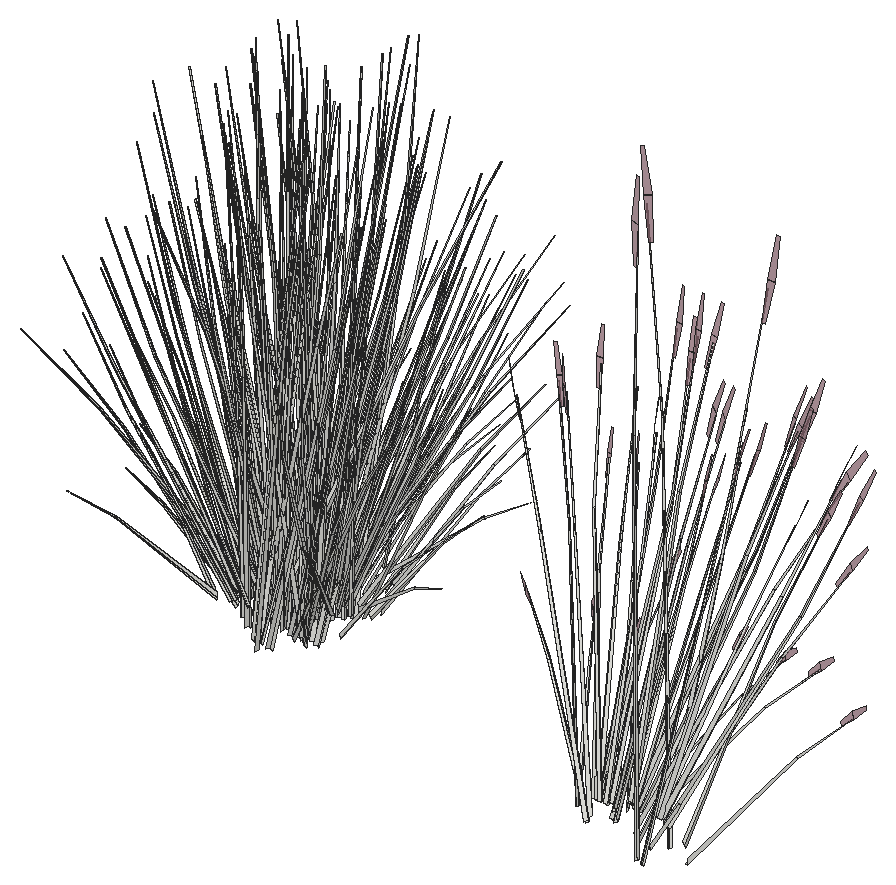
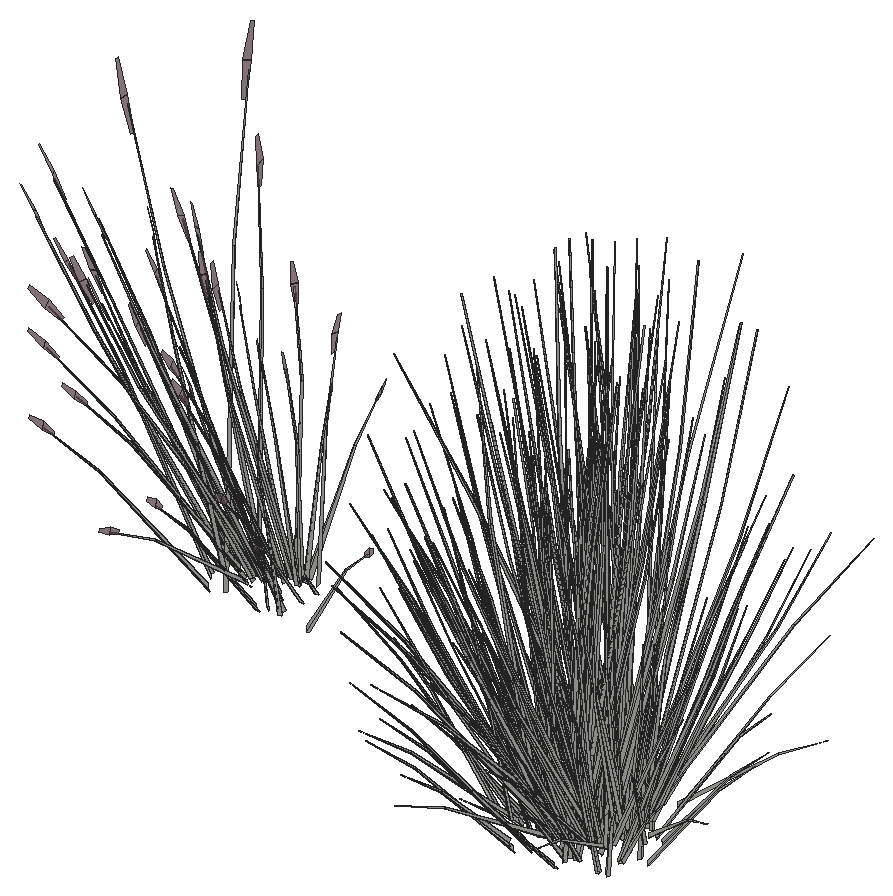
# SketchUp Ruby script. Lengths in inches.
U = 1.inch
M = Sketchup.active_model
def pt(a) = Geom::Point3d.new(a.map { |v| v * U })
def face(e, loops, mat)
  f = e.add_face(loops[0].map { |a| pt(a) })
  loops[1..].each { |l| e.add_face(l.map { |a| pt(a) }).erase! }
  f.material = f.back_material = mat if mat
  f
end
# faces: each face lists its corners as indices into pts; further lists are holes
def faces(e, pts, list, mat = nil) = list.each { |f| face(e, (f[0].is_a?(Array) ? f : [f]).map { |l| l.map { |i| pts[i] } }, mat) }
# xy, xz, yz: faces in a plane at the given z, y or x. An outline is a flat list of corners, or four numbers for a rectangle; further outlines are holes
def ring(l) = l.size == 4 ? [[l[0], l[1]], [l[2], l[1]], [l[2], l[3]], [l[0], l[3]]] : l.each_slice(2).to_a
def flat(e, list, mat, &to3) = list.each { |f| face(e, (f[0].is_a?(Array) ? f : [f]).map { |l| ring(l).map { |u, v| to3.(u, v) } }, mat) }
def xy(e, z, list, mat = nil) = flat(e, list, mat) { |x, y| [x, y, z] }
def xz(e, y, list, mat = nil) = flat(e, list, mat) { |x, z| [x, y, z] }
def yz(e, x, list, mat = nil) = flat(e, list, mat) { |y, z| [x, y, z] }
def lines(e, pts, list) = list.each { |a, b| e.add_line(pt(pts[a]), pt(pts[b])) }
# prism: a flat outline (further loops are holes) pulled along v
def prism(e, loops, v, mat = nil)
  f = face(e, loops, mat); d = Geom::Vector3d.new(v.map { |x| x * U })
  f.pushpull(f.normal.samedirection?(d) ? d.length : -d.length)
end
def box(e, o, s, mat = nil) = prism(e, [[o, [o[0] + s[0], o[1], o[2]], [o[0] + s[0], o[1] + s[1], o[2]], [o[0], o[1] + s[1], o[2]]]], [0, 0, s[2]], mat)
def at(x, y, z, deg = 0) = Geom::Transformation.translation(pt([x, y, z])) * Geom::Transformation.rotation(ORIGIN, Z_AXIS, deg.degrees)
def axes(o, x, y, z) = Geom::Transformation.new([*x, 0, *y, 0, *z, 0, *pt(o).to_a, 1])
def part(name) = M.definitions.add(name)
# library, detail: a bought-in or finely detailed component or shape, given as its bounding box
def library(name, o, s) = part(name).tap { |d| box(d.entities, o, s) }
def detail(e, o, s) = box(e.add_group.entities, o, s)
def put(e, d, t, mat = nil) = e.add_instance(d, t).tap { |i| i.material = mat if mat }
def group(e, t, mat = nil) = e.add_group.tap { |g| g.transformation = t; g.material = mat if mat }.entities
root = M.entities
M.materials.add("LightPink_Translucent").color = [144, 107, 117]
M.materials["LightPink_Translucent"].alpha = 0.75
c1 = part("blade")
p = [[2.15,0.21,22],[0,0.17,0],[0.09,0.45,0],[2.18,0.31,22],[2.29,0.31,22],[0.38,0.45,0],
  [2.48,0.24,33],[2.49,0.24,33],[2.48,0.22,33]]
faces(c1.entities,p,[[0,1,2,3],[4,5,2,3],[6,3,4,7],[8,0,3,6]])
c2 = part("seeds")
p = [[0.3,-0.1,1.38],[-0.01,-0.03,1.59],[-0.01,-0.03,0.03],[0.14,-0.07,-0.07],[0.29,-0.03,3],[0.15,0.01,3.11]]
faces(c2.entities,p,[[0,1,2,3],[1,0,4,5]],"LightPink_Translucent")
c3 = part("blade with seeds")
put(c3.entities,c1,at(0,0,0))
put(c3.entities,c2,axes([2.4,0.25,30.99],[1.5799,-0.05474,1.17369],[-0.12525,1.92788,0.29478],[-0.07173,-0.02425,1.56792]))
c4 = part("blade with seeds\#1")
put(c4.entities,c1,at(0,0,0))
put(root,c3,axes([267.38,266.44,17.27],[0.73026,-0.88648,-0.1216],[1.05755,0.51071,-0.67495],[0.36761,0.25045,1.02557]))
put(root,c4,axes([224.3,276.92,16.28],[-0.8363,-0.68892,-0.10962],[0.4818,-0.99769,-0.60845],[0.23628,-0.3468,0.92453]))
put(root,c3,axes([262.1,263.23,16.11],[0.30609,-0.31822,1.71376],[0.77286,0.85893,0.13857],[-0.53009,0.39116,0.73262]))
put(root,c3,axes([261.13,264.16,16.92],[0.31482,0.94565,-0.51099],[-1.19224,0.16542,-0.3958],[-0.34166,0.254,0.97773]))
put(root,c4,axes([218.74,280.28,13.18],[0.39117,1.13797,1.16227],[-1.12236,0.3622,0.45161],[0.01867,-0.69878,1.32195]))
put(root,c3,axes([262.5625,265.24,17.29],[0.82919,-0.54528,0.35414],[0.78493,0.62262,-0.4572],[-0.11943,0.31634,0.87481]))
put(root,c3,axes([268.77,266.35,14.61],[0.7662,1.03778,0],[-1.28187,0.57875,-0.51607],[-0.29196,0.13181,1.63711]))
put(root,c4,axes([219.2,273.87,16.29],[0.13963,1.00636,0.31925],[-0.79822,0.26574,-0.41216],[-0.2144,-0.28839,0.78863]))
put(root,c3,axes([266.42,267.18,16.95],[0.00363,-0.12539,1.77383],[1.0502,-0.55319,-0.16761],[0.36479,0.19745,0.31391]))
put(root,c4,axes([224.77,274.52,14.14],[-0.03064,0.74138,0.9471],[-0.6508,-0.48961,0.52291],[0.23122,-0.29288,0.74292]))
put(root,c3,axes([270,266.7,13.73],[0.08928,-0.14952,1.76342],[1.12407,-0.44035,-0.26939],[0.34078,0.22791,0.30037]))
put(root,c3,axes([268.12,262.24,15.08],[-0.03348,-0.97511,1.41272],[1.51511,0.25277,0.59816],[-0.35835,0.53357,1.3335]))
put(root,c3,axes([268.51,263.3,14.33],[0.44936,0.94823,-0.69212],[-1.29441,0.3415,-0.18165],[0.04967,0.32109,1.52773]))
put(root,c3,axes([261.8125,265.74,16.97],[-1.00708,-0.04826,0.0643],[0.02761,-0.72867,0.50621],[-0.10538,0.27912,0.77189]))
put(root,c4,axes([216.97,276.76,15.23],[0.33582,0.21526,1.54493],[-0.69497,0.90306,0.12492],[-0.43315,-0.40739,0.66044]))
put(root,c3,axes([259.67,266.57,13.73],[0.16438,0.10347,1.76342],[0.27873,0.95868,-0.26939],[-0.36432,0.20444,0.30037]))
put(root,c3,axes([262.13,265.8,16.97],[-0.87265,-0.70663,0.48003],[0.92674,-0.60943,0.3958],[-0.16097,0.33153,0.9933]))
put(root,c3,axes([268.24,266,16.92],[1.20928,-0.24619,-0.51099],[0.21154,0.93233,-0.3958],[0.32481,0.26718,0.97773]))
put(root,c3,axes([264.89,266.14,17.29],[0.36946,-0.79643,0.35414],[1.07787,0.23229,-0.4572],[0.09883,0.32066,0.87481]))
put(root,c4,axes([220.73,272.66,13.88],[0,-1.44565,0],[1.09198,0,-0.46523],[0.24871,0,1.47583]))
put(root,c4,axes([219.3125,277.33,14.14],[-0.64866,-1.16728,-0.26229],[0.91655,-0.77622,-0.45076],[0.09308,-0.288,1.43974]))
put(root,c4,axes([217.95,274.69,13.57],[0.85134,-0.27158,-0.27926],[0.24175,1.0786,0.27926],[0.09817,-0.21744,1.25283]))
put(root,c3,axes([269.91,266.95,14.9],[-0.78586,-0.03248,1.0506],[0.51898,-0.68985,0.58006],[0.31045,0.24509,0.8241]))
put(root,c4,axes([223.5,274.63,14.23],[-0.28093,0.65095,1.03545],[-0.28545,-0.84053,0.76078],[0.2418,-0.22671,0.22807]))
put(root,c3,axes([267.65,266.76,16.97],[-0.55698,0.6579,0.0643],[-0.79316,-0.38303,0.50621],[0.25643,0.21093,0.77189]))
put(root,c4,axes([216.02,273.57,15.99],[-0.19445,0.01116,1.57709],[-0.562,0.94258,-0.24942],[-0.34067,-0.14573,0.12648]))
put(root,c4,axes([217.08,274.82,16.01],[0.66663,-0.82326,0.43274],[0.57493,0.87428,0.35681],[-0.31276,-0.15186,0.89544]))
put(root,c3,axes([266.34,268.98,17.88],[0.84686,-0.59414,-0.06488],[0.77596,0.65071,-0.29416],[0.05463,0.18438,0.97024]))
put(root,c4,axes([223.2,276.95,14.08],[-0.32388,-0.0204,1.28914],[-0.36177,-0.97496,-0.27724],[0.38765,-0.30097,0.55117]))
put(root,c4,axes([218.61,278.11,13.6],[-0.73437,-0.77871,-0.5621],[0.66591,-0.96736,-0.14753],[-0.18319,-0.31204,1.24074]))
put(root,c4,axes([217.15,274.52,16],[0.04552,-0.95007,0.05797],[0.68742,0.02605,0.45634],[-0.26332,-0.09941,0.69585]))
put(root,c3,axes([267.88,266.58,16.97],[-1.21888,0.23767,0.48003],[-0.21154,-0.93233,0.3958],[0.28666,0.27478,0.9933]))
put(root,c4,axes([219.36,276.14,15.77],[-0.50765,0.99901,1.24659],[-0.79039,-1.05487,0.53787],[0.47632,-0.32232,1.20495]))
put(root,c4,axes([216.88,274.82,15.82],[-0.51441,-0.78225,-0.31925],[0.58738,-0.7405,0.41216],[-0.29843,-0.11267,0.78863]))
put(root,c4,axes([224.99,277.82,15.98],[-0.11829,-0.00342,1.59908],[-0.52187,-0.99076,-0.1511],[0.18628,-0.34414,0.28298]))
put(root,c3,axes([261.87,264.01,16.11],[0.22818,-0.35597,1.71376],[0.95725,0.73667,0.13857],[-0.43183,0.45914,0.73262]))
put(root,c3,axes([267.35,265.27,14.83],[0.02163,-0.34331,1.43002],[1.03345,-0.38348,-0.30754],[0.31903,0.4109,0.61141]))
put(root,c4,axes([223.89,276.82,16.29],[-0.78697,0.17856,0.31925],[-0.2078,-1.02074,-0.41216],[0.22552,-0.27417,0.78863]))
put(root,c4,axes([219.77,276.59,13.73],[0.82007,-0.69452,-0.40331],[0.57748,1.05199,0.1941],[0.10147,-0.22475,1.29492]))
put(root,c3,axes([264.55,266.86,16.97],[-0.90301,0.35198,0.0643],[-0.44199,-0.64184,0.50621],[0.08721,0.28293,0.77189]))
put(root,c3,axes([262.13,266.02,16.76],[-0.82919,0.54528,-0.35414],[-0.78493,-0.62262,0.4572],[-0.11943,0.31634,0.87481]))
put(root,c3,axes([259.27,265.86,16.95],[-0.03046,0.20495,1.74944],[0.86449,0.71297,-0.27667],[-0.22632,0.33716,0.14031]))
put(root,c3,axes([262.04,265.39,17.63],[1.34686,0.05131,-0.13498],[-0.03681,0.97156,-0.74919],[-0.09356,0.37418,1.13838]))
put(root,c3,axes([264.53,266.48,17.27],[1.19922,-0.48218,-0.1216],[0.58932,0.85579,-0.67495],[0.15822,0.36063,1.02557]))
put(root,c3,axes([264.875,266.8,17.3],[-1.20755,-0.27075,0.53283],[0.41292,-0.89013,0.43934],[0.07257,0.35005,1.10256]))
put(root,c3,axes([262.66,268.14,15],[-0.03171,-0.6158,1.1486],[0.7925,0.43922,0.84392],[-0.15586,0.29352,0.25299]))
put(root,c4,axes([217.43,275.34,16.23],[-0.90375,-0.03008,-0.64046],[0.0607,-1.26677,0.07729],[-0.38287,-0.13368,0.906]))
put(root,c4,axes([217.51,275.67,13.97],[-0.48852,1.08202,0.44759],[-0.87598,-0.64674,0],[0.11126,-0.24644,1.41987]))
put(root,c4,axes([222.61,276.62,13.71],[-0.33151,-1.21377,-0.17307],[0.95493,-0.4265,0.00007],[-0.03664,-0.13398,1.56765]))
put(root,c3,axes([264.74,266.66,13.73],[0.19833,-0.05635,1.76342],[1.19302,0.31018,-0.26939],[0.03489,0.3496,0.30037]))
put(root,c4,axes([220.5625,273.54,13.97],[-0.97703,0,0.44759],[0,-1.29348,0],[0.22253,0,1.41987]))
put(root,c3,axes([262.96,265.76,17.24],[0.87728,0.69587,-0.5672],[-0.92674,0.60943,-0.43934],[-0.13348,0.35356,1.08528]))
put(root,c4,axes([219.03,277.22,14.1],[-0.87196,-0.22303,0.13053],[0.15136,-1.08968,-0.37274],[0.08953,-0.19831,1.14258]))
put(root,c4,axes([222.56,277.99,15.23],[-0.31369,0.26428,1.54493],[-0.26409,-1.22118,0.12492],[0.49247,-0.276,0.66044]))
put(root,c4,axes([221.47,272.99,13.56],[0.97703,0,-0.44759],[0,1.29348,0],[0.22253,0,1.41987]))
put(root,c3,axes([262,266.8,15.06],[1.11329,-0.1834,0.06507],[0.25594,0.73887,-0.86304],[-0.07058,0.37403,0.7736]))
put(root,c4,axes([224.43,276.4375,16.01],[0.22422,1.14989,0.43274],[-0.87956,0.19957,0.35681],[0.25922,-0.27044,0.89544]))
put(root,c3,axes([265.56,266.43,16.92],[1.20468,0.25962,-0.51099],[-0.41292,0.89013,-0.3958],[0.11046,0.35838,0.97773]))
put(root,c3,axes([266.24,264.6,16.11],[-0.28013,-0.33252,1.71376],[1.29445,-0.27994,0.13857],[0.29256,0.52202,0.73262]))
put(root,c4,axes([224.6,276.66,16],[0.62066,0.52545,0.05797],[-0.36135,0.74826,0.45634],[0.19899,-0.24191,0.69585]))
put(root,c4,axes([216.6,279.39,13.56],[-0.48852,-1.08202,-0.44759],[0.87598,-0.64674,0],[-0.11126,-0.24644,1.41987]))
put(root,c4,axes([215.96,276.14,14.08],[0.19776,0.32863,1.28914],[-0.34614,0.98419,-0.27724],[-0.43048,-0.18244,0.55117]))
put(root,c3,axes([265.01,266.98,16.76],[-0.36946,0.79643,-0.35414],[-1.07787,-0.23229,0.4572],[0.09883,0.32066,0.87481]))
put(root,c3,axes([262.68,265.44,17.57],[-0.03189,0.95798,-0.7886],[-1.34277,-0.06434,0.09517],[-0.14171,0.40585,1.11556]))
put(root,c3,axes([259.17,267.96,16.95],[0.13903,-0.06253,1.77383],[1.14912,0.41591,-0.16761],[-0.027,0.34629,0.31391]))
put(root,c4,axes([220.34,276.37,14.14],[0.46619,-1.302,-0.26229],[0.98396,0.62692,-0.45076],[0.24158,-0.04092,1.43974]))
put(root,c4,axes([217.125,275.59,15.96],[-0.65648,0.82762,-0.46065],[-0.57493,-0.87428,-0.35681],[-0.33354,-0.12593,0.88141]))
put(root,c4,axes([216.99,279.14,13.57],[0.24175,-1.0786,-0.27926],[0.85134,0.27158,0.27926],[-0.09817,-0.21744,1.25283]))
put(root,c3,axes([263.95,264.76,16.11],[-0.02999,-0.3975,1.71376],[1.30002,0.26369,0.13857],[-0.08041,0.56647,0.73262]))
put(root,c4,axes([219.26,277.69,14.19],[-0.82007,0.69452,0.40331],[-0.57748,-1.05199,-0.1941],[0.10147,-0.22475,1.29492]))
put(root,c4,axes([220.27,276,14.1],[-0.28493,-1.07717,0.13053],[0.81364,-0.37722,-0.37274],[0.17907,0,1.14258]))
put(root,c4,axes([217.61,275.23,16.29],[0.51441,0.78225,0.31925],[-0.58738,0.7405,-0.41216],[-0.29843,-0.11267,0.78863]))
put(root,c4,axes([219.46,278.95,14.14],[-1.11485,0.13472,-0.26229],[-0.06741,-1.40314,-0.45076],[-0.1485,-0.24708,1.43974]))
put(root,c4,axes([221.45,273.54,13.57],[0.60959,0.80703,-0.27926],[-0.60959,0.80703,0.27926],[0.19635,0,1.25283]))
put(root,c4,axes([220.375,276.45,13.73],[0,-1.29348,0],[1.0115,0,0],[0,0,1.60831]))
put(root,c4,axes([217.47,274.73,16.28],[-0.04841,1.27062,-0.10962],[-0.91657,-0.03473,-0.60845],[-0.353,-0.08826,0.92453]))
put(root,c4,axes([221.34,275.85,13.63],[0.89455,-0.42392,-0.62393],[0.32217,1.22114,-0.16376],[0.30292,-0.04686,1.37722]))
put(root,c3,axes([265.12,266.26,17.22],[0.5849,0.8421,-0.71045],[-1.20401,0.4693,0.08574],[0.13677,0.40688,1.00501]))
put(root,c4,axes([215.32,273.82,15.98],[0.07463,0.11741,1.59908],[-0.25178,1.15035,-0.1511],[-0.32567,0.04164,0.28298]))
put(root,c4,axes([219.86,276.86,13.89],[-0.20585,1.46124,0.44352],[-1.16261,-0.29738,0.17404],[0.11226,-0.21355,1.53985]))
put(root,c3,axes([261.73,267.59,14.83],[0.38672,-0.16338,1.43002],[0.95481,0.49262,-0.30754],[-0.28419,0.42626,0.61141]))
put(root,c3,axes([264.24,268.39,16.95],[0.15534,0.16677,1.74944],[1.25362,0.06552,-0.27667],[0.12606,0.3678,0.14031]))
put(root,c4,axes([220.07,276.48,14.19],[-0.88038,-0.56093,0.40331],[0.4237,-1.16553,-0.1941],[0.20294,0,1.29492]))
put(root,c4,axes([224.33,279.6,16.28],[-0.45489,-1.13134,-0.10962],[0.80735,-0.55596,-0.60845],[0.34022,-0.14927,0.92453]))
put(root,c4,axes([224.29,278.63,15.96],[0.24493,-1.13649,-0.46065],[0.83975,0.38955,-0.35681],[0.33809,-0.10421,0.88141]))
put(root,c4,axes([223.13,276.97,13.73],[0.43865,-1.16553,0],[0.91144,0.56093,0],[0,0,1.57718]))
put(root,c4,axes([220.81,276.47,13.74],[0.63109,-0.80703,0],[0.63109,0.80703,0],[0,0,1.52591]))
put(root,c4,axes([221.29,273.24,13.72],[-0.00781,1.44494,-0.04486],[-1.09198,0,0.45022],[0.24858,0.04541,1.42752]))
put(root,c4,axes([226.69,277.89,16.83],[-0.56051,-0.79893,-0.05849],[0.61388,-0.73204,-0.26518],[0.17394,-0.05154,0.87466]))
put(root,c4,axes([219.41,278.11,13.87],[0.88667,0.95859,0.41247],[-0.7827,1.13884,0.16186],[-0.08849,-0.2311,1.43206]))
put(root,c4,axes([218,276.08,13.97],[0.25932,1.24233,0.15904],[-0.96507,0.30677,0.3163],[0.14061,-0.1108,1.44604]))
put(root,c4,axes([214.39,277.35,14.23],[0.56973,-0.14831,1.03545],[-0.31555,0.82274,0.76078],[-0.29172,-0.08853,0.22807]))
put(root,c4,axes([216.75,280.375,13.88],[-0.97904,0.72283,0],[-0.54599,-1.20931,-0.46523],[-0.12435,-0.27543,1.47583]))
put(root,c3,axes([262.23,266.79,15.6],[0.02693,-0.53464,1.54345],[1.21102,0.2824,0.21329],[-0.10493,0.5698,0.72882]))
put(root,c4,axes([224.13,279.05,16.23],[0.79444,-0.5518,-0.64046],[0.44274,1.13586,0.07729],[0.38385,-0.12903,0.906]))
put(root,c4,axes([220.53,274.29,13.97],[-0.71168,0.90835,0.15904],[-0.69029,-0.91538,0.3163],[0.14534,0.10032,1.44604]))
put(root,c4,axes([222.76,277.39,13.8],[1.12244,-0.50265,-0.0542],[0.39331,1.43622,0],[0.0392,-0.01755,1.55211]))
put(root,c4,axes([224.01,279.26,16.29],[-0.75135,-0.34854,0.31925],[0.21915,-1.01686,-0.41216],[0.30251,-0.09324,0.78863]))
put(root,c4,axes([220.125,277.43,13.73],[-1.1305,0,0],[0,-1.44565,0],[0,0,1.61777]))
put(root,c4,axes([219.67,279.19,14.19],[0.06031,1.25545,0.40331],[-1.00118,0.11354,-0.1941],[-0.10147,-0.22475,1.29492]))
put(root,c4,axes([217.95,279.78,13.97],[0.971,0.33398,0.15904],[-0.27478,1.22215,0.3163],[-0.00473,-0.21112,1.44604]))
put(root,c4,axes([220.57,276.7,13.81],[1.12994,0,-0.05082],[0,1.44565,0],[0.03551,0,1.61697]))
put(root,c4,axes([216.15,277.41,16.01],[0.25543,-1.1392,0.43274],[0.83975,0.38955,0.35681],[-0.33023,0.06846,0.89544]))
put(root,c4,axes([216.09,277.1,16],[-0.33205,-0.8519,0.05797],[0.60551,-0.41697,0.45634],[-0.26692,0.08227,0.69585]))
put(root,c4,axes([220.33,278.77,13.93],[0.47355,-1.30265,0.21694],[0.98396,0.62692,0.45076],[-0.22682,0,1.44726]))
put(root,c4,axes([226.14,279.87,15.99],[0.15733,-0.14655,1.57709],[0.06181,-1.18266,-0.24942],[0.34698,-0.11893,0.12648]))
put(root,c4,axes([221.07,276.51,13.73],[0.88038,0.56093,-0.40331],[-0.4237,1.16553,0.1941],[0.20294,0,1.29492]))
put(root,c4,axes([222.73,278.03,13.73],[-0.84234,0.37722,0],[-0.29498,-1.07717,0],[0,0,1.39163]))
put(root,c4,axes([224.51,279.4,13.09],[-0.05317,-0.18711,1.5897],[0.29263,-1.12549,-0.24285],[0.32981,-0.03291,0.27078]))
put(root,c4,axes([215.97,277.53,15.82],[-0.75135,-0.34854,-0.31925],[0.21915,-1.01686,0.41216],[-0.30251,0.09324,0.78863]))
put(root,c4,axes([224.81,279.15,15.82],[0.75135,0.34854,-0.31925],[-0.21915,1.01686,0.41216],[0.30251,-0.09324,0.78863]))
put(root,c4,axes([223.53,275.85,13.97],[-0.48852,-1.08202,0.44759],[0.87598,-0.64674,0],[0.11126,0.24644,1.41987]))
put(root,c4,axes([219.89,279.47,13.73],[-0.88038,-0.56093,-0.40331],[0.4237,-1.16553,0.1941],[-0.20294,0,1.29492]))
put(root,c4,axes([221,277.0625,13.8125],[-0.84094,1.07538,-0.05527],[-0.84146,-1.07603,0],[-0.02937,0.03755,1.58274]))
put(root,c4,axes([223.6,276.48,13.84],[0.31757,-1.44738,0.27726],[1.13512,0.3621,-0.32897],[0.14207,0.23956,1.48641]))
put(root,c4,axes([220.03,279.23,13.87],[1.09253,-0.50265,0.41247],[0.37991,1.43622,0.16186],[-0.20075,-0.01755,1.43206]))
put(root,c4,axes([214.89,278.59,13.09],[0.0352,0.19392,1.5897],[-0.39624,1.07238,-0.24285],[-0.33051,-0.01799,0.27078]))
put(root,c4,axes([223.01,276.2,13.97],[-0.971,-0.33398,0.15904],[0.27478,-1.22215,0.3163],[0.00473,0.21112,1.44604]))
put(root,c4,axes([221.29,276.78,14.19],[-0.06031,-1.25545,0.40331],[1.00118,-0.11354,-0.1941],[0.10147,0.22475,1.29492]))
put(root,c4,axes([221.72,276.76,14.1],[0.58702,-0.85413,0.13053],[0.66228,0.71246,-0.37274],[0.08953,0.19831,1.14258]))
put(root,c4,axes([224.7,279.58,16],[0.33205,0.8519,0.05797],[-0.60551,0.41697,0.45634],[0.26692,-0.08227,0.69585]))
put(root,c4,axes([224.63,279.28,16.3],[-0.25543,1.1392,0.48034],[-0.83975,-0.38955,0.39606],[0.33023,-0.06846,0.99394]))
put(root,c4,axes([223.11,278.29,13.72],[-0.43865,1.16553,0],[-0.91144,-0.56093,0],[0,0,1.46678]))
put(root,c4,axes([224.21,275.6,13.88],[0.97904,-0.72283,0],[0.54599,1.20931,-0.46523],[0.12435,0.27543,1.47583]))
put(root,c4,axes([216.77,277.42,16.29],[0.75135,0.34854,0.31925],[-0.21915,1.01686,-0.41216],[-0.30251,0.09324,0.78863]))
put(root,c4,axes([222.96,279.89,13.97],[-0.25932,-1.24233,0.15904],[0.96507,-0.30677,0.3163],[-0.14061,0.1108,1.44604]))
put(root,c4,axes([216.65,277.64,16.23],[-0.79444,0.5518,-0.64046],[-0.44274,-1.13586,0.07729],[-0.38385,0.12903,0.906]))
put(root,c4,axes([220.89,279.49,14.19],[0.88038,0.56093,0.40331],[-0.4237,1.16553,-0.1941],[-0.20294,0,1.29492]))
put(root,c4,axes([215.57,278.79,13.66],[0.56051,0.79893,-0.03509],[-0.61388,0.73204,-0.15911],[-0.17394,0.05154,0.52479]))
put(root,c4,axes([221.1,279.11,13.87],[0.20585,-1.46124,0.41247],[1.16261,0.29738,0.16186],[-0.11226,0.21355,1.43206]))
put(root,c4,axes([222.71,280.15,15.23],[-0.375,0.0283,1.54493],[0.24877,-1.22643,0.12492],[0.53441,0.07586,0.66044]))
put(root,c4,axes([216.49,278.05,15.96],[-0.24493,1.13649,-0.46065],[-0.83975,-0.38955,-0.35681],[-0.33809,0.10421,0.88141]))
put(root,c4,axes([216.45,277.08,16.28],[0.45489,1.13134,-0.10962],[-0.80735,0.55596,-0.60845],[-0.34022,0.14927,0.92453]))
put(root,c4,axes([219.52,282.43,13.57],[-0.60959,-0.80703,-0.27926],[0.60959,-0.80703,0.27926],[-0.19635,0,1.25283]))
put(root,c4,axes([219.63,280.1875,13.63],[-1.0019,0.47479,-0.62955],[-0.36083,-1.36768,-0.16523],[-0.33927,0.05248,1.38963]))
put(root,c4,axes([221.51,277.02,14.14],[1.11485,-0.13472,-0.26229],[0.06741,1.40314,-0.45076],[0.1485,0.24708,1.43974]))
put(root,c4,axes([220.33,276.21,14.3],[-0.91991,0.03158,1.27354],[0.23846,-1.42935,0.53923],[0.50337,0.33806,1.20213]))
put(root,c4,axes([223.98,276.83,13.57],[-0.24175,1.0786,-0.27926],[-0.85134,-0.27158,0.27926],[0.09817,0.21744,1.25283]))
put(root,c4,axes([224.64,281.99,14.28],[-0.17302,-1.05027,0.05866],[0.69705,-0.24145,-0.77802],[0.35285,0.06658,0.69739]))
put(root,c4,axes([220.625,279.61,14.14],[-0.46619,1.302,-0.26229],[-0.98396,-0.62692,-0.45076],[-0.24158,0.04092,1.43974]))
put(root,c4,axes([223.31,281.95,16.61],[0.04841,-1.27062,-0.12168],[0.91657,0.03473,-0.67538],[0.353,0.08826,1.02623]))
put(root,c4,axes([224.1,276.51,13.72],[-0.98246,0.71382,-0.04636],[-0.54599,-1.20931,0.46523],[0.09354,0.298,1.4751]))
put(root,c4,axes([223.17,281.46,16.29],[-0.51441,-0.78225,0.31925],[0.58738,-0.7405,-0.41216],[0.29843,0.11267,0.78863]))
put(root,c4,axes([224.36,276.58,13.56],[0.48852,1.08202,-0.44759],[-0.87598,0.64674,0],[0.11126,0.24644,1.41987]))
put(root,c4,axes([223.65,281.09,16.25],[0.65648,-0.82762,-0.51132],[0.57493,0.87428,-0.39606],[0.33354,0.12593,0.97836]))
put(root,c4,axes([214.34,278.875,15.99],[-0.13699,0.17683,1.57709],[0.08685,1.18009,-0.24942],[-0.32765,0.18834,0.12648]))
put(root,c4,axes([219.49,282.99,13.56],[-0.97703,0,-0.44759],[0,-1.29348,0],[-0.22253,0,1.41987]))
put(root,c4,axes([221.66,279.28,13.9375],[-1.15773,-0.30643,-0.21121],[0.20181,-1.4529,0.4622],[-0.15988,0.25387,1.41028]))
put(root,c4,axes([221.93,278.75,14.1],[0.87196,0.22303,0.13053],[-0.15136,1.08968,-0.37274],[-0.08953,0.19831,1.14258]))
put(root,c4,axes([220.4,282.43,13.97],[0.97703,0,0.44759],[0,1.29348,0],[-0.22253,0,1.41987]))
put(root,c4,axes([224.63,281.77,14.77],[-0.50438,-0.0254,1.3914],[0.26641,-1.14247,0.19228],[0.53755,0.09899,0.65702]))
put(root,c4,axes([216.18,280.02,16],[-0.62066,-0.52545,0.05797],[0.36135,-0.74826,0.45634],[-0.19899,0.24191,0.69585]))
put(root,c4,axes([221.78,277.9,13.73],[0.06031,1.25545,-0.40331],[-1.00118,0.11354,0.1941],[0.10147,0.22475,1.29492]))
put(root,c4,axes([223.45,280.3,13.97],[0.48852,-1.08202,0.44759],[0.87598,0.64674,0],[-0.11126,0.24644,1.41987]))
put(root,c4,axes([221.94,277.33,13.96],[-0.78639,1.12892,-0.2271],[-0.88305,-0.94994,0.49699],[0.09199,0.304,1.51643]))
put(root,c4,axes([225.9,281.37,14.23],[-0.58095,0.02992,1.03545],[0.41436,-0.74764,0.76078],[0.2769,0.14704,0.22807]))
put(root,c4,axes([221.1875,279.38,13.73],[-0.82007,0.69452,-0.40331],[-0.57748,-1.05199,0.1941],[-0.10147,0.22475,1.29492]))
put(root,c4,axes([215.97,280.32,16.33],[-0.25113,-1.28788,0.48466],[0.9851,-0.22351,0.39963],[-0.29033,0.30289,1.00289]))
put(root,c4,axes([223.35,281.34,16.55],[0.90375,0.03008,-0.71091],[-0.0607,1.26677,0.08579],[0.38287,0.13368,1.00565]))
put(root,c4,axes([222.22,277.76,14.74],[0.39398,-0.99907,1.36359],[0.84877,0.97875,0.53923],[-0.50305,0.4384,1.14314]))
put(root,c4,axes([215.07,281.58,14.23],[0.34005,-0.60308,1.03545],[0.20441,0.87829,0.76078],[-0.26134,0.18792,0.22807]))
put(root,c4,axes([222.36,277.86,13.6],[0.73437,0.77871,-0.5621],[-0.66591,0.96736,-0.14753],[0.18319,0.31204,1.24074]))
put(root,c4,axes([216.89,279.86,16.29],[0.78697,-0.17856,0.31925],[0.2078,1.02074,-0.41216],[-0.22552,0.27417,0.78863]))
put(root,c4,axes([219.95,282.1875,13.84],[0.82143,1.07538,0.27726],[-0.81279,1.07603,-0.32897],[-0.23327,0.03755,1.48641]))
put(root,c4,axes([225.73,284.65,15.98],[-0.05899,-0.13116,1.59908],[0.39237,-1.08407,-0.1511],[0.32669,0.02548,0.28298]))
put(root,c4,axes([223.01,281.28,13.57],[-0.85134,0.27158,-0.27926],[-0.24175,-1.0786,0.27926],[-0.09817,0.21744,1.25283]))
put(root,c4,axes([216.25,280.46,15.82],[-0.78697,0.17856,-0.31925],[-0.2078,-1.02074,0.41216],[-0.22552,0.27417,0.78863]))
put(root,c4,axes([223.9,281.87,15.82],[0.51441,0.78225,-0.31925],[-0.58738,0.7405,0.41216],[0.29843,0.11267,0.78863]))
put(root,c4,axes([223.63,282.17,16],[-0.04552,0.95007,0.05797],[-0.68742,-0.02605,0.45634],[0.26332,0.09941,0.69585]))
put(root,c4,axes([221.65,278.64,14.14],[0.64866,1.16728,-0.26229],[-0.91655,0.77622,-0.45076],[-0.09308,0.288,1.43974]))
put(root,c4,axes([220.23,283.31,13.88],[0,1.44565,0],[-1.09198,0,-0.46523],[-0.24871,0,1.47583]))
put(root,c4,axes([223.7,281.86,16.01],[-0.66663,0.82326,0.43274],[-0.57493,-0.87428,0.35681],[0.31276,0.15186,0.89544]))
put(root,c4,axes([216.42,280.89,15.23],[0.31369,-0.26428,1.54493],[0.26409,1.22118,0.12492],[-0.49247,0.276,0.66044]))
put(root,c4,axes([215.59,281.22,14.08],[0.31962,0.07001,1.28914],[0.26756,1.02347,-0.27724],[-0.41311,0.23924,0.55117]))
put(root,c4,axes([213.89,280.08,15.98],[0.11711,0.02157,1.59908],[0.42502,1.06376,-0.1511],[-0.21726,0.31303,0.28298]))
put(root,c4,axes([225.38,282.24,14.08],[-0.15413,-0.36483,1.28914],[0.46474,-0.90077,-0.27724],[0.40213,0.2681,0.55117]))
put(root,c4,axes([216.59,282.76,13.66],[0.7978,0.33351,-0.03509],[-0.24541,1.02647,-0.15911],[-0.13049,0.15585,0.52479]))
put(root,c4,axes([221.58,282.82,16.29],[-0.13963,-1.00636,0.31925],[0.79822,-0.26574,-0.41216],[0.2144,0.28839,0.78863]))
put(root,c4,axes([223.84,285.1,16.83],[0.2608,-1.0202,-0.05849],[0.8027,0.31383,-0.26518],[0.12187,0.16686,0.87466]))
put(root,c4,axes([223.96,280.92,13.88],[0.97904,0.72283,0],[-0.54599,1.20931,-0.46523],[-0.12435,0.27543,1.47583]))
put(root,c4,axes([223.375,281.58,13.56],[-0.48852,1.08202,-0.44759],[-0.87598,-0.64674,0],[-0.11126,0.24644,1.41987]))
put(root,c4,axes([216.875,280.12,16.23],[-0.47225,0.98582,-0.64046],[-0.82754,-0.7006,0.07729],[-0.28197,0.35717,0.906]))
put(root,c4,axes([216.1,282.05,13.09],[0.12871,0.11199,1.5897],[0.2775,1.13173,-0.24285],[-0.25244,0.2734,0.27078]))
put(root,c4,axes([216.9,280.58,15.96],[0.23225,1.14083,-0.46065],[-0.87956,0.19957,-0.35681],[-0.25205,0.30642,0.88141]))
put(root,c4,axes([221.51,283.34,16.28],[0.53874,-1.06944,-0.10962],[0.78019,0.61612,-0.60845],[0.2712,0.30214,0.92453]))
put(root,c4,axes([221.5,280,13.6],[-0.16018,1.20264,-0.5621],[-0.98808,-0.25378,-0.14753],[-0.11973,0.3589,1.24074]))
put(root,c4,axes([216.11,279.78,16.63],[0.93666,0.77159,-0.12278],[-0.53962,1.11741,-0.68147],[-0.26463,0.38842,1.03548]))
put(root,c4,axes([217.95,281.89,16.29],[0.61172,-0.65782,0.31925],[0.57907,0.75112,-0.41216],[-0.08811,0.38163,0.78863]))
put(root,c4,axes([217.4,282.49,16],[-0.74296,-0.05822,0.05797],[0.02037,-0.87906,0.45634],[-0.07774,0.33673,0.69585]))
put(root,c4,axes([223.75,284.5625,15.99],[0.19335,0.02874,1.57709],[0.67262,-0.81555,-0.24942],[0.31807,0.21351,0.12648]))
put(root,c4,axes([222.14,282.81,15.96],[0.89213,-0.297,-0.46065],[0.15606,1.12475,-0.35681],[0.23962,0.32232,0.88141]))
put(root,c4,axes([219.67,282.98,16.29],[0.27256,-0.96081,0.31925],[0.79518,0.28024,-0.41216],[0.07291,0.38684,0.78863]))
put(root,c4,axes([222,282.11,15.23],[-0.33582,-0.21526,1.54493],[0.69497,-0.90306,0.12492],[0.43315,0.40739,0.66044]))
put(root,c4,axes([221.7,283.73,16],[-0.4109,0.79368,0.05797],[-0.58514,-0.46209,0.45634],[0.18917,0.25446,0.69585]))
put(root,c4,axes([217.4,282.92,16.33],[-0.72104,-0.95477,0.48466],[0.76573,-0.82343,0.39963],[-0.133,0.44794,1.00289]))
put(root,c4,axes([221.88,283.51,16.01],[-0.89921,0.28673,0.43274],[-0.15606,-1.12475,0.35681],[0.21148,0.33149,0.89544]))
put(root,c4,axes([221.26,281.9,15.23],[-0.3002,-0.28876,1.54493],[0.81031,-0.72911,0.12492],[0.36902,0.50009,0.66044]))
put(root,c4,axes([224.42,284.18,13.09],[0.09761,-0.15508,1.5897],[0.90442,-0.26295,-0.24285],[0.19286,0.3437,0.27078]))
put(root,c4,axes([219.1,284.41,14.23],[-0.06991,-0.73811,1.03545],[0.616,0.4682,0.76078],[-0.09241,0.36475,0.22807]))
put(root,c4,axes([217.63,282.83,15.82],[-0.61172,0.65782,-0.31925],[-0.57907,-0.75112,0.41216],[-0.08811,0.38163,0.78863]))
put(root,c4,axes([222.05,283.64,15.82],[0.13963,1.00636,-0.31925],[-0.79822,0.26574,0.41216],[0.2144,0.28839,0.78863]))
put(root,c4,axes([219.42,283.85,16],[-0.66618,0.42462,0.05797],[-0.32607,-0.77431,0.45634],[0.06434,0.34133,0.69585]))
put(root,c4,axes([217.56,282.07,16.28],[0.99362,0.0619,-0.10962],[-0.02716,1.17208,-0.60845],[-0.06902,0.45141,0.92453]))
put(root,c4,axes([219.66,283.76,16.01],[-0.89085,-0.32663,0.43274],[0.30463,-1.07385,0.35681],[0.05354,0.4223,0.89544]))
put(root,c4,axes([219.4,283.38,16.28],[0.88471,-0.5817,-0.10962],[0.43476,1.03242,-0.60845],[0.11673,0.43507,0.92453]))
put(root,c4,axes([215.84,282.74,15.99],[-0.0069,0.24875,1.57709],[0.68965,0.79195,-0.24942],[-0.14092,0.42256,0.12648]))
put(root,c4,axes([223.96,285.45,14.23],[-0.44281,-0.48182,1.03545],[0.70101,-0.19012,0.76078],[0.12552,0.34819,0.22807]))
put(root,c4,axes([216.43,283.7,15.98],[0.0975,-0.08571,1.59908],[0.87648,0.41319,-0.1511],[0.00634,0.41846,0.28298]))
put(root,c4,axes([218.24,282.51,15.96],[0.6472,0.83949,-0.46065],[-0.68369,0.73521,-0.35681],[-0.09847,0.42653,0.88141]))
put(root,c4,axes([220.11,283.87,13.09],[0.15398,-0.02932,1.5897],[0.80412,0.59108,-0.24285],[-0.04053,0.41985,0.27078]))
put(root,c4,axes([220.16,283.33,15.96],[0.88873,0.31321,-0.46065],[-0.30463,1.07385,-0.35681],[0.08149,0.43235,0.88141]))
put(root,c4,axes([221.22,286.69,15.98],[0.0262,-0.14755,1.59908],[0.86326,-0.45644,-0.1511],[0.22658,0.30203,0.28298]))
put(root,c4,axes([219.76,283.99,15.82],[-0.27256,0.96081,-0.31925],[-0.79518,-0.28024,0.41216],[0.07291,0.38684,0.78863]))
put(root,c4,axes([217.39,282.66,15.23],[0.16834,-0.42944,1.54493],[0.70619,0.88871,0.12492],[-0.31858,0.5539,0.66044]))
put(root,c4,axes([218.04,282.13,16.23],[-0.02352,1.1557,-0.64046],[-0.99061,-0.07762,0.07729],[-0.10454,0.48961,0.906]))
put(root,c4,axes([218.28,283.0625,14.08],[0.27202,-0.22572,1.28914],[0.7394,0.52014,-0.27724],[-0.17673,0.53408,0.55117]))
put(root,c4,axes([220.29,284.59,15.99],[0.12685,0.18879,1.57709],[0.92682,-0.01606,-0.24942],[0.12053,0.43275,0.12648]))
put(root,c4,axes([219.625,281.0625,14.75],[-0.14134,-0.32863,1.5962],[0.98684,-0.11332,0.12492],[0.13095,0.71181,0.57049]))
put(root,c4,axes([222.25,284.62,14.08],[0.08021,-0.40179,1.28914],[0.81924,-0.25896,-0.27724],[0.15335,0.54576,0.55117]))
put(root,c4,axes([220.62,283.37,15.23],[-0.20666,-0.40114,1.54493],[0.95496,-0.33772,0.12492],[0.21583,0.62976,0.66044]))
put(root,c4,axes([218.93,283.57,15.23],[-0.02213,-0.47954,1.54493],[0.95907,0.31812,0.12492],[-0.05932,0.68338,0.66044]))
